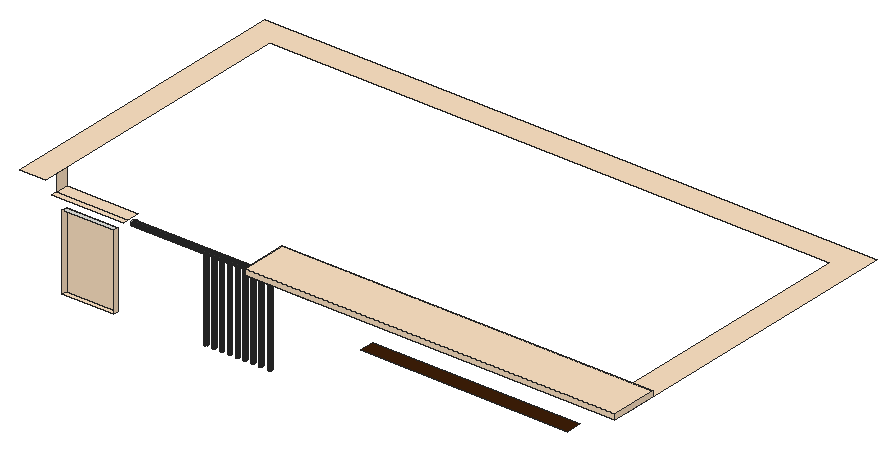
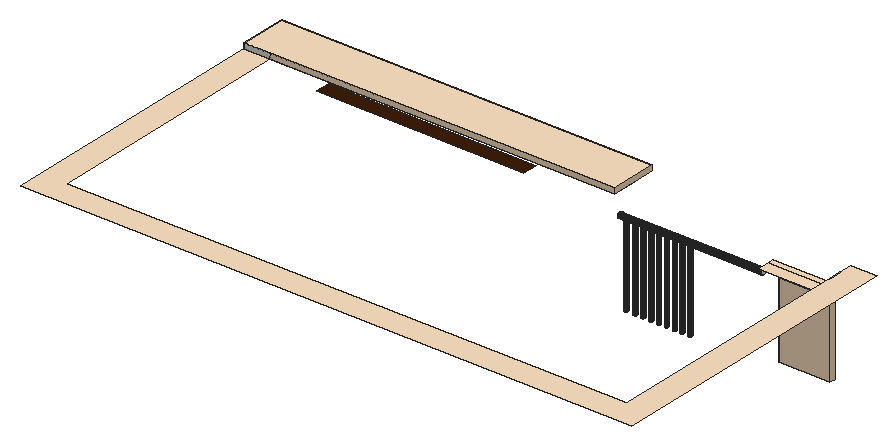
# SketchUp Ruby script. Lengths in inches.
U = 1.inch
M = Sketchup.active_model
def pt(a) = Geom::Point3d.new(a.map { |v| v * U })
def face(e, loops, mat)
  f = e.add_face(loops[0].map { |a| pt(a) })
  loops[1..].each { |l| e.add_face(l.map { |a| pt(a) }).erase! }
  f.material = f.back_material = mat if mat
  f
end
# faces: each face lists its corners as indices into pts; further lists are holes
def faces(e, pts, list, mat = nil) = list.each { |f| face(e, (f[0].is_a?(Array) ? f : [f]).map { |l| l.map { |i| pts[i] } }, mat) }
# xy, xz, yz: faces in a plane at the given z, y or x. An outline is a flat list of corners, or four numbers for a rectangle; further outlines are holes
def ring(l) = l.size == 4 ? [[l[0], l[1]], [l[2], l[1]], [l[2], l[3]], [l[0], l[3]]] : l.each_slice(2).to_a
def flat(e, list, mat, &to3) = list.each { |f| face(e, (f[0].is_a?(Array) ? f : [f]).map { |l| ring(l).map { |u, v| to3.(u, v) } }, mat) }
def xy(e, z, list, mat = nil) = flat(e, list, mat) { |x, y| [x, y, z] }
def xz(e, y, list, mat = nil) = flat(e, list, mat) { |x, z| [x, y, z] }
def yz(e, x, list, mat = nil) = flat(e, list, mat) { |y, z| [x, y, z] }
def lines(e, pts, list) = list.each { |a, b| e.add_line(pt(pts[a]), pt(pts[b])) }
# prism: a flat outline (further loops are holes) pulled along v
def prism(e, loops, v, mat = nil)
  f = face(e, loops, mat); d = Geom::Vector3d.new(v.map { |x| x * U })
  f.pushpull(f.normal.samedirection?(d) ? d.length : -d.length)
end
def box(e, o, s, mat = nil) = prism(e, [[o, [o[0] + s[0], o[1], o[2]], [o[0] + s[0], o[1] + s[1], o[2]], [o[0], o[1] + s[1], o[2]]]], [0, 0, s[2]], mat)
def at(x, y, z, deg = 0) = Geom::Transformation.translation(pt([x, y, z])) * Geom::Transformation.rotation(ORIGIN, Z_AXIS, deg.degrees)
def axes(o, x, y, z) = Geom::Transformation.new([*x, 0, *y, 0, *z, 0, *pt(o).to_a, 1])
def part(name) = M.definitions.add(name)
# library, detail: a bought-in or finely detailed component or shape, given as its bounding box
def library(name, o, s) = part(name).tap { |d| box(d.entities, o, s) }
def detail(e, o, s) = box(e.add_group.entities, o, s)
def put(e, d, t, mat = nil) = e.add_instance(d, t).tap { |i| i.material = mat if mat }
def group(e, t, mat = nil) = e.add_group.tap { |g| g.transformation = t; g.material = mat if mat }.entities
root = M.entities
M.materials.add("[0012_Bisque]").color = [255, 228, 196]
M.materials.add("[0043_SaddleBrown]").color = [63, 31, 8]
M.materials.add("[Color M07]").color = [58, 58, 58]
xy(root,297.36,[[28.1875,180.33,68.35,184.58]],"[0012_Bisque]")
xy(root,352.96,[[276.43,162.83,439.49,174.45]],"[0043_SaddleBrown]")
xy(root,356.45,[[28.1875,180.33,68.35,184.58]])
xy(root,359.5625,[[103.26,188.34,103.61,188.39,103.94,188.53,104.23,188.75,104.45,189.03,104.58,189.36,104.63,189.72,104.58,190.07,104.45,190.41,104.23,190.69,103.94,190.91,103.61,191.05,103.26,191.09,102.9,191.05,102.57,190.91,102.28,190.69,102.06,190.41,101.93,190.07,101.88,189.72,101.93,189.36,102.06,189.03,102.28,188.75,102.57,188.53,102.9,188.39]])
xy(root,359.6875,[[158.38,188.34,158.74,188.39,159.07,188.53,159.35,188.75,159.57,189.03,159.71,189.36,159.76,189.72,159.71,190.07,159.57,190.41,159.35,190.69,159.07,190.91,158.74,191.05,158.38,191.09,158.02,191.05,157.69,190.91,157.41,190.69,157.19,190.41,157.05,190.07,157.01,189.72,157.05,189.36,157.19,189.03,157.41,188.75,157.69,188.53,158.02,188.39]])
xy(root,359.9375,[[109.38,188.34,109.74,188.39,110.07,188.53,110.35,188.75,110.57,189.03,110.71,189.36,110.76,189.72,110.71,190.07,110.57,190.41,110.35,190.69,110.07,190.91,109.74,191.05,109.38,191.09,109.02,191.05,108.69,190.91,108.41,190.69,108.19,190.41,108.05,190.07,108.01,189.72,108.05,189.36,108.19,189.03,108.41,188.75,108.69,188.53,109.02,188.39],[127.76,188.34,128.11,188.39,128.44,188.53,128.73,188.75,128.95,189.03,129.08,189.36,129.13,189.72,129.08,190.07,128.95,190.41,128.73,190.69,128.44,190.91,128.11,191.05,127.76,191.09,127.4,191.05,127.07,190.91,126.78,190.69,126.56,190.41,126.43,190.07,126.38,189.72,126.43,189.36,126.56,189.03,126.78,188.75,127.07,188.53,127.4,188.39]])
xy(root,359.95,[[121.63,188.34,121.99,188.39,122.32,188.53,122.6,188.75,122.82,189.03,122.96,189.36,123.01,189.72,122.96,190.07,122.82,190.41,122.6,190.69,122.32,190.91,121.99,191.05,121.63,191.09,121.27,191.05,120.94,190.91,120.66,190.69,120.44,190.41,120.3,190.07,120.26,189.72,120.3,189.36,120.44,189.03,120.66,188.75,120.94,188.53,121.27,188.39]])
xy(root,360,[[133.88,188.34,134.24,188.39,134.57,188.53,134.85,188.75,135.07,189.03,135.21,189.36,135.26,189.72,135.21,190.07,135.07,190.41,134.85,190.69,134.57,190.91,134.24,191.05,133.88,191.09,133.52,191.05,133.19,190.91,132.91,190.69,132.69,190.41,132.55,190.07,132.51,189.72,132.55,189.36,132.69,189.03,132.91,188.75,133.19,188.53,133.52,188.39]])
xy(root,360.125,[[78.76,188.34,79.11,188.39,79.44,188.53,79.73,188.75,79.95,189.03,80.08,189.36,80.13,189.72,80.08,190.07,79.95,190.41,79.73,190.69,79.44,190.91,79.11,191.05,78.76,191.09,78.4,191.05,78.07,190.91,77.78,190.69,77.56,190.41,77.43,190.07,77.38,189.72,77.43,189.36,77.56,189.03,77.78,188.75,78.07,188.53,78.4,188.39]])
xy(root,360.1875,[[84.88,188.34,85.24,188.39,85.57,188.53,85.85,188.75,86.07,189.03,86.21,189.36,86.26,189.72,86.21,190.07,86.07,190.41,85.85,190.69,85.57,190.91,85.24,191.05,84.88,191.09,84.52,191.05,84.19,190.91,83.91,190.69,83.69,190.41,83.55,190.07,83.51,189.72,83.55,189.36,83.69,189.03,83.91,188.75,84.19,188.53,84.52,188.39],[176.82,188.34,177.17,188.39,177.51,188.53,177.79,188.75,178.01,189.03,178.15,189.36,178.19,189.72,178.15,190.07,178.01,190.41,177.79,190.69,177.51,190.91,177.17,191.05,176.82,191.09,176.46,191.05,176.13,190.91,175.85,190.69,175.63,190.41,175.49,190.07,175.44,189.72,175.49,189.36,175.63,189.03,175.85,188.75,176.13,188.53,176.46,188.39]])
xy(root,360.3125,[[97.13,188.34,97.49,188.39,97.82,188.53,98.1,188.75,98.32,189.03,98.46,189.36,98.51,189.72,98.46,190.07,98.32,190.41,98.1,190.69,97.82,190.91,97.49,191.05,97.13,191.09,96.77,191.05,96.44,190.91,96.16,190.69,95.94,190.41,95.8,190.07,95.76,189.72,95.8,189.36,95.94,189.03,96.16,188.75,96.44,188.53,96.77,188.39]])
xy(root,360.375,[[170.63,188.34,170.99,188.39,171.32,188.53,171.6,188.75,171.82,189.03,171.96,189.36,172.01,189.72,171.96,190.07,171.82,190.41,171.6,190.69,171.32,190.91,170.99,191.05,170.63,191.09,170.27,191.05,169.94,190.91,169.66,190.69,169.44,190.41,169.3,190.07,169.26,189.72,169.3,189.36,169.44,189.03,169.66,188.75,169.94,188.53,170.27,188.39]])
xy(root,360.625,[[152.26,188.34,152.61,188.39,152.94,188.53,153.23,188.75,153.45,189.03,153.58,189.36,153.63,189.72,153.58,190.07,153.45,190.41,153.23,190.69,152.94,190.91,152.61,191.05,152.26,191.09,151.9,191.05,151.57,190.91,151.28,190.69,151.06,190.41,150.93,190.07,150.88,189.72,150.93,189.36,151.06,189.03,151.28,188.75,151.57,188.53,151.9,188.39]])
xy(root,360.6875,[[140.01,188.34,140.36,188.39,140.69,188.53,140.98,188.75,141.2,189.03,141.33,189.36,141.38,189.72,141.33,190.07,141.2,190.41,140.98,190.69,140.69,190.91,140.36,191.05,140.01,191.09,139.65,191.05,139.32,190.91,139.03,190.69,138.81,190.41,138.68,190.07,138.63,189.72,138.68,189.36,138.81,189.03,139.03,188.75,139.32,188.53,139.65,188.39]])
xy(root,360.8125,[[146.13,188.34,146.49,188.39,146.82,188.53,147.1,188.75,147.32,189.03,147.46,189.36,147.51,189.72,147.46,190.07,147.32,190.41,147.1,190.69,146.82,190.91,146.49,191.05,146.13,191.09,145.77,191.05,145.44,190.91,145.16,190.69,144.94,190.41,144.8,190.07,144.76,189.72,144.8,189.36,144.94,189.03,145.16,188.75,145.44,188.53,145.77,188.39]])
xy(root,361.02,[[91.01,188.34,91.36,188.39,91.69,188.53,91.98,188.75,92.2,189.03,92.33,189.36,92.38,189.72,92.33,190.07,92.2,190.41,91.98,190.69,91.69,190.91,91.36,191.05,91.01,191.09,90.65,191.05,90.32,190.91,90.03,190.69,89.81,190.41,89.68,190.07,89.63,189.72,89.68,189.36,89.81,189.03,90.03,188.75,90.32,188.53,90.65,188.39],[115.51,188.34,115.86,188.39,116.19,188.53,116.48,188.75,116.7,189.03,116.83,189.36,116.88,189.72,116.83,190.07,116.7,190.41,116.48,190.69,116.19,190.91,115.86,191.05,115.51,191.09,115.15,191.05,114.82,190.91,114.53,190.69,114.31,190.41,114.18,190.07,114.13,189.72,114.18,189.36,114.31,189.03,114.53,188.75,114.82,188.53,115.15,188.39],[164.51,188.34,164.86,188.39,165.19,188.53,165.48,188.75,165.7,189.03,165.83,189.36,165.88,189.72,165.83,190.07,165.7,190.41,165.48,190.69,165.19,190.91,164.86,191.05,164.51,191.09,164.15,191.05,163.82,190.91,163.53,190.69,163.31,190.41,163.18,190.07,163.13,189.72,163.18,189.36,163.31,189.03,163.53,188.75,163.82,188.53,164.15,188.39],[184.01,188.34,184.36,188.39,184.69,188.53,184.98,188.75,185.2,189.03,185.33,189.36,185.38,189.72,185.33,190.07,185.2,190.41,184.98,190.69,184.69,190.91,184.36,191.05,184.01,191.09,183.65,191.05,183.32,190.91,183.03,190.69,182.81,190.41,182.68,190.07,182.63,189.72,182.68,189.36,182.81,189.03,183.03,188.75,183.32,188.53,183.65,188.39]])
xy(root,364.375,[[20.26,180.33,76.27,184.58],[20.26,184.58,76.27,194.72]],"[0012_Bisque]")
xy(root,377.375,[[189.35,162.83,206.61,174.45],[209.66,162.83,224.17,174.45],[227.22,162.83,241.23,174.45],[244.28,162.83,257.3,174.45],[260.36,162.83,439.49,174.45],
  [439.49,162.83,480,174.45],[189.35,174.45,480,194.72]])
xy(root,377.375,[[189.35,158.14,206.61,162.83],[206.61,158.14,209.66,174.45],[209.66,158.14,224.17,162.83],[224.17,158.14,227.22,174.45],[227.22,158.14,241.23,162.83],
  [241.23,158.14,244.28,174.45],[244.28,158.14,257.3,162.83],[257.3,158.14,260.36,174.45],[260.36,158.14,439.49,162.83],[439.49,158.14,480,162.83],
  [0,174.45,20.26,174.45,20.26,394.19,459.74,394.19,459.74,194.72,480,194.72,480,414.45,0,414.45]],"[0012_Bisque]")
xy(root,381.75,[[189.35,158.14,480,194.72]],"[0012_Bisque]")
xz(root,158.14,[[189.35,377.375,480,381.75]],"[0012_Bisque]")
xz(root,184.58,[[28.1875,297.36,68.35,356.45]],"[0012_Bisque]")
xz(root,194.72,[[459.74,377.375,480,381.75]])
xz(root,194.72,[[189.35,377.375,459.74,381.75]],"[0012_Bisque]")
yz(root,20.26,[[184.58,364.375,194.72,377.375]],"[0012_Bisque]")
yz(root,28.1875,[[180.33,297.36,184.58,356.45]],"[0012_Bisque]")
yz(root,68.35,[[180.33,297.36,184.58,356.45]],"[0012_Bisque]")
yz(root,76.27,[[189.8125,358.43,189.28,358.5,188.78,358.7,188.35,359.03,188.02,359.46,187.82,359.95,187.75,360.49,187.82,361.02,188.02,361.52,188.35,361.95,188.78,362.27,189.28,362.48,189.8125,362.55,190.34,362.48,190.84,362.27,191.27,361.95,191.6,361.52,191.8,361.02,191.875,360.49,191.8,359.95,191.6,359.46,191.27,359.03,190.84,358.7,190.34,358.5]])
yz(root,189.35,[[158.14,377.375,194.72,381.75]],"[0012_Bisque]")
yz(root,480,[[158.14,377.375,194.72,381.75]],"[0012_Bisque]")
p = [[133.52,188.39,295],[133.88,188.34,295],[133.88,188.34,360],[133.52,188.39,360],[134.24,188.39,295],[134.24,188.39,360],
  [139.65,188.39,295],[140.01,188.34,295],[140.01,188.34,360.6875],[139.65,188.39,360.6875],[140.36,188.39,295],[140.36,188.39,360.6875],
  [145.77,188.39,295],[146.13,188.34,295],[146.13,188.34,360.8125],[145.77,188.39,360.8125],[146.49,188.39,295],[146.49,188.39,360.8125],
  [151.9,188.39,295],[152.26,188.34,295],[152.26,188.34,360.625],[151.9,188.39,360.625],[152.61,188.39,295],[152.61,188.39,360.625],
  [158.02,188.39,295],[158.38,188.34,295],[158.38,188.34,359.6875],[158.02,188.39,359.6875],[158.74,188.39,295],[158.74,188.39,359.6875],
  [164.15,188.39,295],[164.51,188.34,295],[164.51,188.34,361.02],[164.15,188.39,361.02],[164.86,188.39,295],[164.86,188.39,361.02],
  [170.27,188.39,295],[170.63,188.34,295],[170.63,188.34,360.375],[170.27,188.39,360.375],[170.99,188.39,295],[170.99,188.39,360.375],
  [176.46,188.39,295],[176.82,188.34,295],[176.82,188.34,360.1875],[176.46,188.39,360.1875],[177.17,188.39,295],[177.17,188.39,360.1875],
  [183.65,188.39,295],[184.01,188.34,295],[184.01,188.34,361.02],[183.65,188.39,361.02],[184.36,188.39,295],[184.36,188.39,361.02],
  [133.19,188.53,295],[133.19,188.53,360],[134.57,188.53,295],[134.57,188.53,360],[139.32,188.53,295],[139.32,188.53,360.6875],
  [140.69,188.53,295],[140.69,188.53,360.6875],[145.44,188.53,295],[145.44,188.53,360.8125],[146.82,188.53,295],[146.82,188.53,360.8125],
  [151.57,188.53,295],[151.57,188.53,360.625],[152.94,188.53,295],[152.94,188.53,360.625],[157.69,188.53,295],[157.69,188.53,359.6875],
  [159.07,188.53,295],[159.07,188.53,359.6875],[163.82,188.53,295],[163.82,188.53,361.02],[165.19,188.53,295],[165.19,188.53,361.02],
  [169.94,188.53,295],[169.94,188.53,360.375],[171.32,188.53,295],[171.32,188.53,360.375],[176.13,188.53,295],[176.13,188.53,360.1875],
  [177.51,188.53,295],[177.51,188.53,360.1875],[183.32,188.53,295],[183.32,188.53,361.02],[184.69,188.53,295],[184.69,188.53,361.02],
  [132.91,188.75,295],[132.91,188.75,360],[139.03,188.75,295],[139.03,188.75,360.6875],[140.98,188.75,295],[140.98,188.75,360.6875],
  [145.16,188.75,295],[145.16,188.75,360.8125],[147.1,188.75,295],[147.1,188.75,360.8125],[151.28,188.75,295],[151.28,188.75,360.625],
  [153.23,188.75,295],[153.23,188.75,360.625],[157.41,188.75,295],[157.41,188.75,359.6875],[159.35,188.75,295],[159.35,188.75,359.6875],
  [163.53,188.75,295],[163.53,188.75,361.02],[165.48,188.75,295],[165.48,188.75,361.02],[169.66,188.75,295],[169.66,188.75,360.375],
  [171.6,188.75,295],[171.6,188.75,360.375],[175.85,188.75,295],[175.85,188.75,360.1875],[177.79,188.75,295],[177.79,188.75,360.1875],
  [183.03,188.75,295],[183.03,188.75,361.02],[184.98,188.75,295],[184.98,188.75,361.02],[132.69,189.03,295],[132.69,189.03,360],
  [138.81,189.03,295],[138.81,189.03,360.6875],[141.2,189.03,295],[141.2,189.03,360.6875],[144.94,189.03,295],[144.94,189.03,360.8125],
  [147.32,189.03,295],[147.32,189.03,360.8125],[151.06,189.03,295],[151.06,189.03,360.625],[153.45,189.03,295],[153.45,189.03,360.625],
  [157.19,189.03,295],[157.19,189.03,359.6875],[159.57,189.03,295],[159.57,189.03,359.6875],[163.31,189.03,295],[163.31,189.03,361.02],
  [165.7,189.03,295],[165.7,189.03,361.02],[169.44,189.03,295],[169.44,189.03,360.375],[171.82,189.03,295],[171.82,189.03,360.375],
  [175.63,189.03,295],[175.63,189.03,360.1875],[178.01,189.03,295],[178.01,189.03,360.1875],[182.81,189.03,295],[182.81,189.03,361.02],
  [185.2,189.03,295],[185.2,189.03,361.02],[132.55,189.36,295],[132.55,189.36,360],[138.68,189.36,295],[138.68,189.36,360.6875],
  [141.33,189.36,295],[141.33,189.36,360.6875],[144.8,189.36,295],[144.8,189.36,360.8125],[147.46,189.36,295],[147.46,189.36,360.8125],
  [150.93,189.36,295],[150.93,189.36,360.625],[153.58,189.36,295],[153.58,189.36,360.625],[157.05,189.36,295],[157.05,189.36,359.6875],
  [159.71,189.36,295],[159.71,189.36,359.6875],[163.18,189.36,295],[163.18,189.36,361.02],[165.83,189.36,295],[165.83,189.36,361.02],
  [169.3,189.36,295],[169.3,189.36,360.375],[171.96,189.36,295],[171.96,189.36,360.375],[175.49,189.36,295],[175.49,189.36,360.1875],
  [178.15,189.36,295],[178.15,189.36,360.1875],[182.68,189.36,295],[182.68,189.36,361.02],[185.33,189.36,295],[185.33,189.36,361.02],
  [132.51,189.72,295],[132.51,189.72,360],[135.21,189.36,295],[135.26,189.72,295],[135.26,189.72,360],[135.21,189.36,360],
  [138.63,189.72,295],[138.63,189.72,360.6875],[141.38,189.72,295],[141.38,189.72,360.6875],[144.76,189.72,295],[144.76,189.72,360.8125],
  [147.51,189.72,295],[147.51,189.72,360.8125],[150.88,189.72,295],[150.88,189.72,360.625],[153.63,189.72,295],[153.63,189.72,360.625],
  [157.01,189.72,295],[157.01,189.72,359.6875],[159.76,189.72,295],[159.76,189.72,359.6875],[163.13,189.72,295],[163.13,189.72,361.02],
  [165.88,189.72,295],[165.88,189.72,361.02],[169.26,189.72,295],[169.26,189.72,360.375],[172.01,189.72,295],[172.01,189.72,360.375],
  [175.44,189.72,295],[175.44,189.72,360.1875],[178.19,189.72,295],[178.19,189.72,360.1875],[182.63,189.72,295],[182.63,189.72,361.02],
  [185.38,189.72,295],[185.38,189.72,361.02],[132.55,190.07,295],[132.55,190.07,360],[135.21,190.07,295],[135.21,190.07,360],
  [138.68,190.07,295],[138.68,190.07,360.6875],[141.33,190.07,295],[141.33,190.07,360.6875],[144.8,190.07,295],[144.8,190.07,360.8125],
  [147.46,190.07,295],[147.46,190.07,360.8125],[150.93,190.07,295],[150.93,190.07,360.625],[153.58,190.07,295],[153.58,190.07,360.625],
  [157.05,190.07,295],[157.05,190.07,359.6875],[159.71,190.07,295],[159.71,190.07,359.6875],[163.18,190.07,295],[163.18,190.07,361.02],
  [165.83,190.07,295],[165.83,190.07,361.02],[169.3,190.07,295],[169.3,190.07,360.375],[171.96,190.07,295],[171.96,190.07,360.375],
  [175.49,190.07,295],[175.49,190.07,360.1875],[178.15,190.07,295],[178.15,190.07,360.1875],[182.68,190.07,295],[182.68,190.07,361.02],
  [185.33,190.07,295],[185.33,190.07,361.02],[132.69,190.41,295],[132.69,190.41,360],[135.07,190.41,295],[135.07,190.41,360],
  [138.81,190.41,295],[138.81,190.41,360.6875],[141.2,190.41,295],[141.2,190.41,360.6875],[144.94,190.41,295],[144.94,190.41,360.8125],
  [147.32,190.41,295],[147.32,190.41,360.8125],[151.06,190.41,295],[151.06,190.41,360.625],[153.45,190.41,295],[153.45,190.41,360.625],
  [157.19,190.41,295],[157.19,190.41,359.6875],[159.57,190.41,295],[159.57,190.41,359.6875],[163.31,190.41,295],[163.31,190.41,361.02],
  [165.7,190.41,295],[165.7,190.41,361.02],[169.44,190.41,295],[169.44,190.41,360.375],[171.82,190.41,295],[171.82,190.41,360.375],
  [175.63,190.41,295],[175.63,190.41,360.1875],[178.01,190.41,295],[178.01,190.41,360.1875],[182.81,190.41,295],[182.81,190.41,361.02],
  [185.2,190.41,295],[185.2,190.41,361.02],[132.91,190.69,295],[132.91,190.69,360],[134.85,190.69,295],[134.85,190.69,360],
  [139.03,190.69,295],[139.03,190.69,360.6875],[140.98,190.69,295],[140.98,190.69,360.6875],[145.16,190.69,295],[145.16,190.69,360.8125],
  [147.1,190.69,295],[147.1,190.69,360.8125],[151.28,190.69,295],[151.28,190.69,360.625],[153.23,190.69,295],[153.23,190.69,360.625],
  [157.41,190.69,295],[157.41,190.69,359.6875],[159.35,190.69,295],[159.35,190.69,359.6875],[163.53,190.69,295],[163.53,190.69,361.02],
  [165.48,190.69,295],[165.48,190.69,361.02],[169.66,190.69,295],[169.66,190.69,360.375],[171.6,190.69,295],[171.6,190.69,360.375],
  [175.85,190.69,295],[175.85,190.69,360.1875],[177.79,190.69,295],[177.79,190.69,360.1875],[183.03,190.69,295],[183.03,190.69,361.02],
  [184.98,190.69,295],[184.98,190.69,361.02],[133.19,190.91,295],[133.19,190.91,360],[134.57,190.91,295],[134.57,190.91,360],
  [139.32,190.91,295],[139.32,190.91,360.6875],[140.69,190.91,295],[140.69,190.91,360.6875],[145.44,190.91,295],[145.44,190.91,360.8125],
  [146.82,190.91,295],[146.82,190.91,360.8125],[151.57,190.91,295],[151.57,190.91,360.625],[152.94,190.91,295],[152.94,190.91,360.625],
  [157.69,190.91,295],[157.69,190.91,359.6875],[159.07,190.91,295],[159.07,190.91,359.6875],[163.82,190.91,295],[163.82,190.91,361.02],
  [165.19,190.91,295],[165.19,190.91,361.02],[169.94,190.91,295],[169.94,190.91,360.375],[171.32,190.91,295],[171.32,190.91,360.375],
  [176.13,190.91,295],[176.13,190.91,360.1875],[177.51,190.91,295],[177.51,190.91,360.1875],[183.32,190.91,295],[183.32,190.91,361.02],
  [184.69,190.91,295],[184.69,190.91,361.02],[133.52,191.05,295],[133.52,191.05,360],[134.24,191.05,295],[134.24,191.05,360],
  [139.65,191.05,295],[139.65,191.05,360.6875],[140.36,191.05,295],[140.36,191.05,360.6875],[145.77,191.05,295],[145.77,191.05,360.8125],
  [146.49,191.05,295],[146.49,191.05,360.8125],[151.9,191.05,295],[151.9,191.05,360.625],[152.61,191.05,295],[152.61,191.05,360.625],
  [158.02,191.05,295],[158.02,191.05,359.6875],[158.74,191.05,295],[158.74,191.05,359.6875],[164.15,191.05,295],[164.15,191.05,361.02],
  [164.86,191.05,295],[164.86,191.05,361.02],[170.27,191.05,295],[170.27,191.05,360.375],[170.99,191.05,295],[170.99,191.05,360.375],
  [176.46,191.05,295],[176.46,191.05,360.1875],[177.17,191.05,295],[177.17,191.05,360.1875],[183.65,191.05,295],[183.65,191.05,361.02],
  [184.36,191.05,295],[184.36,191.05,361.02],[133.88,191.09,295],[133.88,191.09,360],[140.01,191.09,295],[140.01,191.09,360.6875],
  [146.13,191.09,295],[146.13,191.09,360.8125],[152.26,191.09,295],[152.26,191.09,360.625],[158.38,191.09,295],[158.38,191.09,359.6875],
  [164.51,191.09,295],[164.51,191.09,361.02],[170.63,191.09,295],[170.63,191.09,360.375],[176.82,191.09,295],[176.82,191.09,360.1875],
  [184.01,191.09,295],[184.01,191.09,361.02],[76.27,189.28,358.5],[76.27,189.8125,358.43],[189.35,189.8125,358.43],[189.35,189.28,358.5],
  [76.27,190.34,358.5],[189.35,190.34,358.5],[76.27,188.78,358.7],[189.35,188.78,358.7],[76.27,190.84,358.7],[189.35,190.84,358.7],
  [76.27,188.35,359.03],[189.35,188.35,359.03],[76.27,191.27,359.03],[189.35,191.27,359.03],[76.27,188.02,359.46],[189.35,188.02,359.46],
  [76.27,191.6,359.46],[189.35,191.6,359.46],[76.27,187.82,359.95],[189.35,187.82,359.95],[76.27,191.8,359.95],[189.35,191.8,359.95],
  [76.27,187.75,360.49],[189.35,187.75,360.49],[76.27,191.875,360.49],[189.35,191.875,360.49],[76.27,187.82,361.02],[189.35,187.82,361.02],
  [76.27,191.8,361.02],[189.35,191.8,361.02],[76.27,188.02,361.52],[189.35,188.02,361.52],[76.27,191.6,361.52],[189.35,191.6,361.52],
  [76.27,188.35,361.95],[189.35,188.35,361.95],[76.27,191.27,361.95],[189.35,191.27,361.95],[76.27,188.78,362.27],[189.35,188.78,362.27],
  [76.27,190.84,362.27],[189.35,190.84,362.27],[76.27,189.28,362.48],[189.35,189.28,362.48],[76.27,190.34,362.48],[189.35,190.34,362.48],
  [76.27,189.8125,362.55],[189.35,189.8125,362.55]]
faces(root,p,[[0,1,2,3],[1,4,5,2],[6,7,8,9],[7,10,11,8],[12,13,14,15],[13,16,17,14],[18,19,20,21],[19,22,23,20],
  [24,25,26,27],[25,28,29,26],[30,31,32,33],[31,34,35,32],[36,37,38,39],[37,40,41,38],[42,43,44,45],[43,46,47,44],
  [48,49,50,51],[49,52,53,50],[54,0,3,55],[4,56,57,5],[58,6,9,59],[10,60,61,11],[62,12,15,63],[16,64,65,17],
  [66,18,21,67],[22,68,69,23],[70,24,27,71],[28,72,73,29],[74,30,33,75],[34,76,77,35],[78,36,39,79],[40,80,81,41],
  [82,42,45,83],[46,84,85,47],[86,48,51,87],[52,88,89,53],[90,54,55,91],[92,58,59,93],[60,94,95,61],[96,62,63,97],
  [64,98,99,65],[100,66,67,101],[68,102,103,69],[104,70,71,105],[72,106,107,73],[108,74,75,109],[76,110,111,77],[112,78,79,113],
  [80,114,115,81],[116,82,83,117],[84,118,119,85],[120,86,87,121],[88,122,123,89],[124,90,91,125],[126,92,93,127],[94,128,129,95],
  [130,96,97,131],[98,132,133,99],[134,100,101,135],[102,136,137,103],[138,104,105,139],[106,140,141,107],[142,108,109,143],[110,144,145,111],
  [146,112,113,147],[114,148,149,115],[150,116,117,151],[118,152,153,119],[154,120,121,155],[122,156,157,123],[158,124,125,159],[160,126,127,161],
  [128,162,163,129],[164,130,131,165],[132,166,167,133],[168,134,135,169],[136,170,171,137],[172,138,139,173],[140,174,175,141],[176,142,143,177],
  [144,178,179,145],[180,146,147,181],[148,182,183,149],[184,150,151,185],[152,186,187,153],[188,154,155,189],[156,190,191,157],[192,158,159,193],
  [194,195,196,197],[198,160,161,199],[162,200,201,163],[202,164,165,203],[166,204,205,167],[206,168,169,207],[170,208,209,171],[210,172,173,211],
  [174,212,213,175],[214,176,177,215],[178,216,217,179],[218,180,181,219],[182,220,221,183],[222,184,185,223],[186,224,225,187],[226,188,189,227],
  [190,228,229,191],[230,192,193,231],[195,232,233,196],[234,198,199,235],[200,236,237,201],[238,202,203,239],[204,240,241,205],[242,206,207,243],
  [208,244,245,209],[246,210,211,247],[212,248,249,213],[250,214,215,251],[216,252,253,217],[254,218,219,255],[220,256,257,221],[258,222,223,259],
  [224,260,261,225],[262,226,227,263],[228,264,265,229],[266,230,231,267],[232,268,269,233],[270,234,235,271],[236,272,273,237],[274,238,239,275],
  [240,276,277,241],[278,242,243,279],[244,280,281,245],[282,246,247,283],[248,284,285,249],[286,250,251,287],[252,288,289,253],[290,254,255,291],
  [256,292,293,257],[294,258,259,295],[260,296,297,261],[298,262,263,299],[264,300,301,265],[302,266,267,303],[268,304,305,269],[306,270,271,307],
  [272,308,309,273],[310,274,275,311],[276,312,313,277],[314,278,279,315],[280,316,317,281],[318,282,283,319],[284,320,321,285],[322,286,287,323],
  [288,324,325,289],[326,290,291,327],[292,328,329,293],[330,294,295,331],[296,332,333,297],[334,298,299,335],[300,336,337,301],[338,302,303,339],
  [304,340,341,305],[342,306,307,343],[308,344,345,309],[346,310,311,347],[312,348,349,313],[350,314,315,351],[316,352,353,317],[354,318,319,355],
  [320,356,357,321],[358,322,323,359],[324,360,361,325],[362,326,327,363],[328,364,365,329],[366,330,331,367],[332,368,369,333],[370,334,335,371],
  [336,372,373,337],[374,338,339,375],[340,376,377,341],[378,342,343,379],[344,380,381,345],[382,346,347,383],[348,384,385,349],[386,350,351,387],
  [352,388,389,353],[390,354,355,391],[356,392,393,357],[394,358,359,395],[360,396,397,361],[398,362,363,399],[364,400,401,365],[402,366,367,403],
  [368,404,405,369],[406,370,371,407],[372,408,409,373],[410,374,375,411],[376,410,411,377],[412,378,379,413],[380,412,413,381],[414,382,383,415],
  [384,414,415,385],[416,386,387,417],[388,416,417,389],[418,390,391,419],[392,418,419,393],[420,394,395,421],[396,420,421,397],[422,398,399,423],
  [400,422,423,401],[424,402,403,425],[404,424,425,405],[426,406,407,427],[408,426,427,409],[428,429,430,431],[429,432,433,430],[434,428,431,435],
  [432,436,437,433],[438,434,435,439],[436,440,441,437],[442,438,439,443],[440,444,445,441],[446,442,443,447],[444,448,449,445],[450,446,447,451],
  [448,452,453,449],[454,450,451,455],[452,456,457,453],[458,454,455,459],[456,460,461,457],[462,458,459,463],[460,464,465,461],[466,462,463,467],
  [464,468,469,465],[470,466,467,471],[468,472,473,469],[474,470,471,475],[472,474,475,473]],"[Color M07]")
